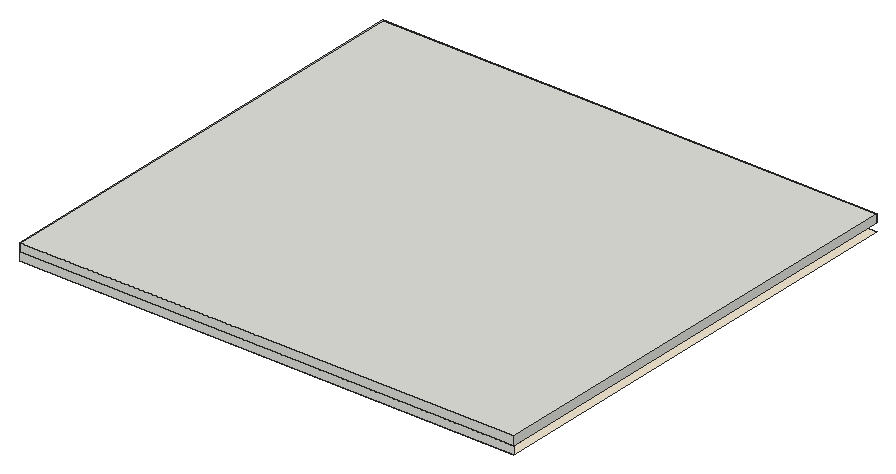
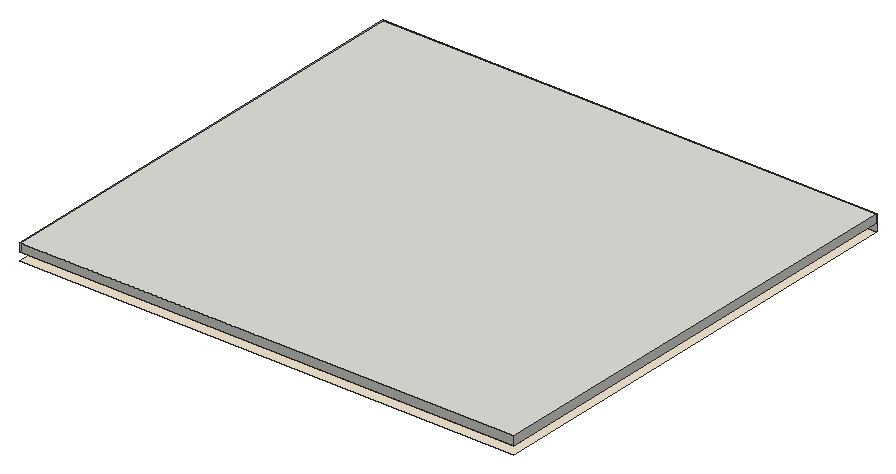
# SketchUp Ruby script. Lengths in inches.
U = 1.inch
M = Sketchup.active_model
def pt(a) = Geom::Point3d.new(a.map { |v| v * U })
def face(e, loops, mat)
  f = e.add_face(loops[0].map { |a| pt(a) })
  loops[1..].each { |l| e.add_face(l.map { |a| pt(a) }).erase! }
  f.material = f.back_material = mat if mat
  f
end
# faces: each face lists its corners as indices into pts; further lists are holes
def faces(e, pts, list, mat = nil) = list.each { |f| face(e, (f[0].is_a?(Array) ? f : [f]).map { |l| l.map { |i| pts[i] } }, mat) }
# xy, xz, yz: faces in a plane at the given z, y or x. An outline is a flat list of corners, or four numbers for a rectangle; further outlines are holes
def ring(l) = l.size == 4 ? [[l[0], l[1]], [l[2], l[1]], [l[2], l[3]], [l[0], l[3]]] : l.each_slice(2).to_a
def flat(e, list, mat, &to3) = list.each { |f| face(e, (f[0].is_a?(Array) ? f : [f]).map { |l| ring(l).map { |u, v| to3.(u, v) } }, mat) }
def xy(e, z, list, mat = nil) = flat(e, list, mat) { |x, y| [x, y, z] }
def xz(e, y, list, mat = nil) = flat(e, list, mat) { |x, z| [x, y, z] }
def yz(e, x, list, mat = nil) = flat(e, list, mat) { |y, z| [x, y, z] }
def lines(e, pts, list) = list.each { |a, b| e.add_line(pt(pts[a]), pt(pts[b])) }
# prism: a flat outline (further loops are holes) pulled along v
def prism(e, loops, v, mat = nil)
  f = face(e, loops, mat); d = Geom::Vector3d.new(v.map { |x| x * U })
  f.pushpull(f.normal.samedirection?(d) ? d.length : -d.length)
end
def box(e, o, s, mat = nil) = prism(e, [[o, [o[0] + s[0], o[1], o[2]], [o[0] + s[0], o[1] + s[1], o[2]], [o[0], o[1] + s[1], o[2]]]], [0, 0, s[2]], mat)
def at(x, y, z, deg = 0) = Geom::Transformation.translation(pt([x, y, z])) * Geom::Transformation.rotation(ORIGIN, Z_AXIS, deg.degrees)
def axes(o, x, y, z) = Geom::Transformation.new([*x, 0, *y, 0, *z, 0, *pt(o).to_a, 1])
def part(name) = M.definitions.add(name)
# library, detail: a bought-in or finely detailed component or shape, given as its bounding box
def library(name, o, s) = part(name).tap { |d| box(d.entities, o, s) }
def detail(e, o, s) = box(e.add_group.entities, o, s)
def put(e, d, t, mat = nil) = e.add_instance(d, t).tap { |i| i.material = mat if mat }
def group(e, t, mat = nil) = e.add_group.tap { |g| g.transformation = t; g.material = mat if mat }.entities
root = M.entities
M.materials.add("0961 AP 7892 PALE IVORY").color = [243, 232, 209]
xy(root,113.78,[[[12,0,198,171],[75.91,7.74,74.64,7.91,73.6,8.09,72.57,8.29,71.54,8.52,70.52,8.79,69.51,9.08,68.5,9.4,67.51,9.75,66.53,10.13,65.56,10.53,64.6,10.97,63.65,11.43,62.72,11.92,61.8,12.44,60.9,12.98,60.01,13.55,59.14,14.15,58.29,14.77,57.45,15.41,56.64,16.08,55.84,16.77,55.07,17.48,54.32,18.22,53.58,18.98,52.875,19.76,52.1875,20.56,51.52,21.375,50.88,22.21,50.27,23.07,49.68,23.9375,49.12,24.83,48.58,25.73,48.07,26.66,47.58,27.59,47.12,28.54,46.69,29.5,46.29,30.48,45.92,31.46,45.57,32.46,45.26,33.46,44.97,34.48,44.71,35.5,44.49,36.53,44.29,37.5625,44.12,38.6,43.99,39.65,43.88,40.69,43.8,41.74,43.76,42.8,43.74,43.82,43.74,129.03,43.76,130.04,43.8,131.07,43.88,132.1,43.99,133.13,44.13,134.16,44.3,135.18,44.5,136.2,44.74,137.21,45,138.21,45.29,139.2,45.61,140.18,45.97,141.16,46.35,142.12,46.76,143.07,47.2,144.01,47.66,144.93,48.16,145.84,48.68,146.74,49.23,147.62,49.8,148.48,50.41,149.32,51.03,150.15,51.68,150.95,52.36,151.74,53.05,152.5,53.77,153.25,54.52,153.97,55.28,154.67,56.07,155.34,56.87,156,57.7,156.62,58.54,157.22,59.4,157.8,60.28,158.35,61.17,158.875,62.08,159.37,63,159.84,63.94,160.28,64.89,160.69,65.85,161.07,66.83,161.43,67.81,161.75,68.8,162.05,69.8,162.31,70.8125,162.54,71.83,162.75,72.85,162.92,73.875,163.0625,74.9,163.17,76.04,163.26,158.18,163.26,159.32,163.16,160.35,163.05,161.37,162.9,162.38,162.72,163.39,162.51,164.39,162.27,165.39,162,166.375,161.7,167.35,161.375,168.32,161.02,169.28,160.63,170.22,160.22,171.15,159.77,172.07,159.3,172.97,158.8,173.86,158.28,174.73,157.73,175.59,157.15,176.42,156.54,177.24,155.92,178.04,155.26,178.82,154.59,179.58,153.89,180.3125,153.17,181.03,152.43,181.72,151.66,182.39,150.875,183.03,150.07,183.65,149.25,184.25,148.41,184.82,147.55,185.36,146.67,185.88,145.78,186.37,144.87,186.83,143.95,187.27,143.02,187.68,142.07,188.05,141.11,188.4,140.14,188.72,139.16,189.01,138.17,189.27,137.17,189.5,136.17,189.7,135.15,189.875,134.14,190.01,133.11,190.12,132.09,190.2,131.0625,190.24,130.03,190.26,129.03,190.26,42.89,190.24,41.88,190.2,40.84,190.12,39.8,190.02,38.77,189.88,37.74,189.71,36.71,189.51,35.69,189.29,34.68,189.03,33.67,188.74,32.67,188.42,31.68,188.08,30.7,187.7,29.73,187.3,28.77,186.87,27.82,186.41,26.89,185.93,25.97,185.42,25.0625,184.88,24.17,184.3125,23.3,183.72,22.44,183.11,21.61,182.47,20.79,181.8,19.98,181.12,19.2,180.41,18.44,179.68,17.7,178.92,16.99,178.15,16.29,177.36,15.62,176.54,14.97,175.71,14.35,174.86,13.75,173.99,13.17,173.11,12.625,172.21,12.1,171.3,11.61,170.37,11.14,169.43,10.7,168.47,10.29,167.51,9.9,166.53,9.55,165.54,9.22,164.54,8.92,163.54,8.65,162.53,8.41,161.51,8.21,160.48,8.03,159.45,7.88,158.24,7.74]],[[75.95,8.37,158.21,8.37,159.375,8.5,160.38,8.65,161.39,8.82,162.39,9.03,163.39,9.26,164.37,9.53,165.35,9.82,166.32,10.14,167.28,10.49,168.23,10.87,169.17,11.27,170.09,11.71,171,12.17,171.9,12.65,172.79,13.17,173.65,13.7,174.51,14.27,175.34,14.86,176.16,15.47,176.96,16.11,177.74,16.77,178.5,17.45,179.24,18.15,179.95,18.88,180.65,19.625,181.33,20.39,181.98,21.18,182.6,21.99,183.21,22.81,183.79,23.65,184.34,24.51,184.87,25.38,185.375,26.27,185.85,27.17,186.3,28.09,186.73,29.02,187.12,29.96,187.49,30.92,187.83,31.88,188.14,32.85,188.42,33.83,188.67,34.82,188.9,35.82,189.09,36.82,189.26,37.83,189.39,38.84,189.5,39.86,189.57,40.88,189.62,41.9,189.63,42.89,189.63,129.03,189.62,130.01,189.57,131.02,189.49,132.03,189.39,133.04,189.25,134.04,189.08,135.04,188.89,136.03,188.66,137.02,188.41,138,188.12,138.97,187.81,139.93,187.46,140.89,187.09,141.83,186.69,142.76,186.27,143.68,185.8125,144.58,185.33,145.47,184.82,146.35,184.29,147.21,183.73,148.05,183.15,148.875,182.54,149.68,181.9,150.47,181.25,151.25,180.57,152,179.86,152.72,179.14,153.43,178.4,154.12,177.63,154.78,176.85,155.42,176.05,156.04,175.22,156.63,174.39,157.2,173.53,157.74,172.66,158.26,171.77,158.74,170.87,159.21,169.96,159.64,169.03,160.05,168.09,160.43,167.14,160.78,166.19,161.1,165.22,161.4,164.24,161.66,163.25,161.9,162.26,162.1,161.27,162.28,160.26,162.42,159.26,162.54,158.15,162.63,76.0625,162.63,74.96,162.55,73.95,162.4375,72.94,162.3,71.94,162.13,70.95,161.93,69.95,161.7,68.97,161.4375,68,161.15,67.03,160.83,66.08,160.48,65.13,160.11,64.2,159.7,63.28,159.27,62.37,158.8125,61.48,158.33,60.6,157.8125,59.74,157.27,58.9,156.71,58.07,156.12,57.26,155.5,56.47,154.86,55.7,154.2,54.95,153.51,54.22,152.8,53.51,152.07,52.83,151.32,52.17,150.55,51.53,149.76,50.91,148.95,50.32,148.12,49.76,147.28,49.22,146.41,48.71,145.53,48.22,144.64,47.76,143.73,47.33,142.8125,46.93,141.88,46.56,140.93,46.21,139.98,45.89,139.01,45.61,138.04,45.35,137.05,45.12,136.0625,44.92,135.07,44.75,134.0625,44.62,133.06,44.51,132.05,44.43,131.03,44.39,130.02,44.37,129.03,44.37,43.82,44.39,42.82,44.43,41.78,44.51,40.75,44.61,39.72,44.75,38.69,44.91,37.67,45.1,36.65,45.33,35.64,45.58,34.64,45.86,33.64,46.17,32.65,46.51,31.68,46.88,30.71,47.27,29.75,47.69,28.81,48.14,27.87,48.62,26.95,49.125,26.05,49.65,25.16,50.21,24.28,50.79,23.43,51.39,22.59,52.02,21.76,52.67,20.96,53.35,20.17,54.04,19.41,54.76,18.66,55.5,17.94,56.26,17.24,57.05,16.56,57.85,15.9,58.67,15.27,59.5,14.66,60.36,14.08,61.23,13.52,62.12,12.98,63.02,12.48,63.93,11.99,64.86,11.54,65.81,11.11,66.76,10.71,67.73,10.34,68.7,10,69.69,9.68,70.69,9.39,71.6875,9.14,72.7,8.91,73.71,8.71,74.73,8.54],[76.02,9.37,74.88,9.53,73.89,9.69,72.9,9.88,71.92,10.11,70.95,10.36,69.98,10.64,69.02,10.94,68.07,11.28,67.14,11.64,66.21,12.03,65.29,12.44,64.39,12.89,63.5,13.35,62.62,13.85,61.76,14.37,60.91,14.91,60.08,15.48,59.27,16.07,58.47,16.6875,57.69,17.32,56.93,17.98,56.19,18.67,55.47,19.37,54.77,20.09,54.09,20.84,53.4375,21.6,52.81,22.38,52.19,23.18,51.61,24,51.04,24.83,50.5,25.68,49.99,26.55,49.5,27.43,49.04,28.32,48.6,29.23,48.19,30.15,47.81,31.08,47.45,32.02,47.12,32.97,46.82,33.93,46.55,34.9,46.3,35.87,46.08,36.85,45.89,37.84,45.74,38.84,45.6,39.83,45.5,40.84,45.43,41.84,45.39,42.84,45.37,43.83,45.37,129.02,45.39,129.99,45.43,130.97,45.5,131.96,45.61,132.9375,45.74,133.91,45.91,134.89,46.1,135.85,46.32,136.82,46.57,137.77,46.85,138.72,47.16,139.65,47.49,140.58,47.85,141.5,48.25,142.4,48.66,143.3,49.11,144.18,49.58,145.04,50.08,145.9,50.6,146.73,51.15,147.55,51.72,148.36,52.31,149.14,52.93,149.91,53.58,150.66,54.24,151.39,54.93,152.1,55.64,152.78,56.36,153.45,57.11,154.09,57.88,154.71,58.66,155.3125,59.47,155.88,60.28,156.43,61.12,156.96,61.97,157.46,62.84,157.93,63.72,158.375,64.61,158.79,65.52,159.19,66.43,159.55,67.36,159.89,68.3,160.2,69.24,160.48,70.2,160.73,71.16,160.95,72.125,161.14,73.1,161.31,74.07,161.44,75.05,161.55,76.1,161.63,158.11,161.63,159.16,161.54,160.14,161.43,161.11,161.29,162.08,161.12,163.04,160.92,163.99,160.69,164.94,160.44,165.88,160.15,166.8125,159.84,167.73,159.5,168.64,159.13,169.54,158.73,170.43,158.3125,171.3,157.86,172.16,157.39,173.01,156.89,173.84,156.36,174.65,155.8125,175.45,155.24,176.23,154.64,176.99,154.02,177.73,153.375,178.45,152.71,179.15,152.02,179.84,151.3125,180.49,150.58,181.13,149.84,181.75,149.07,182.34,148.29,182.9,147.48,183.45,146.67,183.97,145.83,184.46,144.98,184.93,144.12,185.37,143.24,185.78,142.35,186.17,141.45,186.53,140.53,186.86,139.61,187.17,138.68,187.44,137.73,187.69,136.78,187.91,135.83,188.1,134.86,188.26,133.89,188.39,132.92,188.5,131.94,188.57,130.96,188.62,129.98,188.63,129.02,188.63,42.9,188.62,41.93,188.57,40.9375,188.5,39.95,188.4,38.96,188.27,37.98,188.11,37,187.92,36.02,187.7,35.06,187.45,34.1,187.18,33.14,186.88,32.2,186.55,31.26,186.19,30.34,185.81,29.42,185.4,28.52,184.96,27.63,184.5,26.75,184.01,25.89,183.5,25.04,182.96,24.21,182.39,23.39,181.81,22.59,181.2,21.81,180.5625,21.04,179.91,20.3,179.23,19.57,178.54,18.87,177.82,18.18,177.08,17.52,176.32,16.88,175.55,16.26,174.75,15.67,173.94,15.09,173.11,14.55,172.27,14.02,171.41,13.53,170.54,13.05,169.66,12.61,168.76,12.1875,167.85,11.79,166.92,11.43,165.99,11.09,165.05,10.77,164.1,10.49,163.14,10.23,162.18,10.01,161.2,9.81,160.23,9.64,159.25,9.5,158.15,9.37]],[[76.09,10.37,158.09,10.37,159.12,10.49,160.07,10.625,161.02,10.79,161.96,10.98,162.9,11.2,163.83,11.45,164.75,11.73,165.66,12.03,166.57,12.36,167.46,12.72,168.35,13.1,169.22,13.51,170.08,13.9375,170.92,14.4,171.76,14.88,172.57,15.39,173.38,15.92,174.16,16.47,174.93,17.05,175.6875,17.65,176.42,18.27,177.14,18.92,177.83,19.58,178.51,20.27,179.17,20.97,179.8,21.69,180.42,22.43,181.01,23.19,181.58,23.97,182.125,24.76,182.65,25.57,183.15,26.39,183.62,27.23,184.07,28.08,184.49,28.95,184.89,29.82,185.26,30.71,185.61,31.61,185.93,32.52,186.22,33.43,186.49,34.36,186.73,35.29,186.9375,36.23,187.12,37.17,187.28,38.125,187.4,39.08,187.5,40.04,187.57,41,187.62,41.96,187.63,42.91,187.63,129.01,187.62,129.95,187.57,130.9,187.5,131.85,187.4,132.8,187.27,133.74,187.12,134.68,186.93,135.62,186.72,136.54,186.48,137.47,186.21,138.38,185.92,139.28,185.59,140.18,185.24,141.07,184.87,141.94,184.47,142.8,184.04,143.66,183.59,144.49,183.11,145.32,182.61,146.125,182.08,146.92,181.53,147.7,180.96,148.46,180.36,149.2,179.74,149.92,179.1,150.63,178.44,151.32,177.76,151.98,177.0625,152.63,176.34,153.25,175.61,153.85,174.85,154.43,174.08,154.99,173.29,155.52,172.49,156.03,171.67,156.52,170.83,156.98,169.99,157.41,169.125,157.82,168.25,158.21,167.37,158.5625,166.48,158.89,165.58,159.2,164.67,159.47,163.75,159.72,162.82,159.94,161.89,160.14,160.95,160.3,160.01,160.4375,159.0625,160.55,158.07,160.63,76.14,160.63,75.15,160.55,74.2,160.45,73.25,160.32,72.31,160.16,71.37,159.97,70.4375,159.76,69.51,159.51,68.59,159.24,67.6875,158.94,66.79,158.62,65.9,158.26,65.02,157.88,64.16,157.48,63.3,157.04,62.46,156.58,61.64,156.1,60.83,155.59,60.03,155.0625,59.26,154.51,58.49,153.93,57.75,153.33,57.03,152.7,56.32,152.06,55.64,151.39,54.97,150.7,54.33,150,53.7,149.27,53.1,148.53,52.52,147.76,51.97,146.99,51.4375,146.19,50.93,145.38,50.45,144.55,49.99,143.71,49.5625,142.86,49.16,141.99,48.78,141.12,48.43,140.23,48.1,139.33,47.8,138.42,47.53,137.5,47.29,136.58,47.08,135.64,46.89,134.71,46.73,133.76,46.6,132.82,46.5,131.86,46.43,130.91,46.39,129.96,46.37,129.01,46.37,43.84,46.39,42.875,46.43,41.9,46.5,40.92,46.6,39.95,46.72,38.98,46.88,38.02,47.0625,37.06,47.27,36.1,47.51,35.15,47.78,34.21,48.07,33.28,48.39,32.36,48.74,31.44,49.11,30.54,49.51,29.65,49.93,28.77,50.38,27.9,50.86,27.05,51.36,26.21,51.88,25.38,52.43,24.57,53,23.78,53.59,23,54.21,22.24,54.84,21.5,55.5,20.78,56.18,20.07,56.88,19.39,57.6,18.73,58.34,18.09,59.09,17.47,59.87,16.87,60.66,16.3,61.46,15.74,62.29,15.22,63.12,14.71,63.97,14.23,64.84,13.78,65.72,13.35,66.61,12.95,67.51,12.57,68.42,12.22,69.34,11.89,70.27,11.59,71.21,11.32,72.16,11.08,73.11,10.86,74.07,10.67,75.03,10.51],[76.16,11.37,75.18,11.5,74.25,11.66,73.32,11.84,72.39,12.05,71.48,12.29,70.5625,12.55,69.66,12.84,68.77,13.15,67.88,13.5,67.01,13.86,66.14,14.25,65.29,14.67,64.45,15.11,63.625,15.58,62.8125,16.07,62.02,16.58,61.23,17.11,60.47,17.67,59.71,18.25,58.98,18.85,58.27,19.47,57.57,20.12,56.89,20.78,56.23,21.46,55.59,22.16,54.97,22.88,54.375,23.62,53.8,24.37,53.25,25.14,52.72,25.93,52.21,26.73,51.72,27.54,51.26,28.37,50.83,29.21,50.42,30.07,50.03,30.93,49.67,31.8125,49.33,32.7,49.02,33.59,48.74,34.5,48.48,35.41,48.25,36.33,48.04,37.26,47.86,38.1875,47.71,39.125,47.59,40.07,47.49,41.01,47.43,41.95,47.39,42.9,47.37,43.85,47.37,129,47.39,129.93,47.43,130.85,47.5,131.77,47.59,132.7,47.72,133.61,47.875,134.53,48.05,135.43,48.26,136.34,48.5,137.23,48.76,138.12,49.05,139,49.36,139.87,49.7,140.73,50.07,141.58,50.46,142.42,50.88,143.25,51.32,144.0625,51.79,144.86,52.28,145.65,52.79,146.42,53.33,147.17,53.89,147.91,54.47,148.63,55.07,149.33,55.7,150.02,56.34,150.68,57.01,151.33,57.69,151.95,58.39,152.56,59.11,153.14,59.85,153.7,60.6,154.24,61.37,154.75,62.16,155.25,62.96,155.71,63.77,156.16,64.6,156.58,65.43,156.97,66.28,157.34,67.14,157.68,68.01,158,68.89,158.29,69.78,158.55,70.68,158.79,71.58,159,72.49,159.18,73.4,159.33,74.32,159.46,75.24,159.56,76.18,159.63,158.03,159.63,158.96,159.55,159.88,159.45,160.79,159.3125,161.7,159.15,162.6,158.97,163.5,158.75,164.39,158.51,165.27,158.25,166.15,157.95,167.01,157.63,167.87,157.29,168.71,156.91,169.54,156.52,170.36,156.1,171.17,155.65,171.96,155.18,172.74,154.6875,173.51,154.17,174.25,153.63,174.99,153.07,175.7,152.49,176.4,151.88,177.07,151.26,177.73,150.61,178.375,149.95,178.99,149.26,179.59,148.5625,180.17,147.84,180.72,147.11,181.25,146.35,181.76,145.59,182.25,144.8,182.71,144,183.15,143.19,183.57,142.37,183.96,141.53,184.32,140.6875,184.66,139.83,184.97,138.96,185.26,138.08,185.51,137.2,185.75,136.31,185.95,135.41,186.13,134.5,186.28,133.59,186.41,132.68,186.51,131.76,186.57,130.84,186.62,129.92,186.63,129,186.63,42.92,186.62,41.99,186.58,41.06,186.51,40.125,186.41,39.2,186.29,38.27,186.14,37.35,185.96,36.43,185.76,35.52,185.52,34.62,185.27,33.72,184.98,32.83,184.67,31.95,184.34,31.08,183.98,30.22,183.59,29.375,183.18,28.54,182.74,27.71,182.28,26.9,181.8,26.1,181.29,25.32,180.76,24.55,180.21,23.8,179.64,23.06,179.04,22.34,178.43,21.64,177.79,20.96,177.13,20.29,176.46,19.65,175.76,19.03,175.05,18.42,174.32,17.84,173.58,17.28,172.8125,16.75,172.04,16.23,171.24,15.74,170.44,15.27,169.61,14.83,168.78,14.41,167.9375,14.01,167.08,13.64,166.21,13.29,165.34,12.98,164.45,12.68,163.56,12.41,162.65,12.17,161.75,11.96,160.83,11.77,159.91,11.61,158.99,11.48,158.04,11.37]]],"0961 AP 7892 PALE IVORY")
xy(root,116.78,[[12,0,198,171]],"0961 AP 7892 PALE IVORY")
xy(root,120,[[12,0,198,171]])
xz(root,0,[[12,113.78,198,116.78],[12,116.78,198,120]])
xz(root,11.37,[[76.16,113.78,158.04,115.78]],"0961 AP 7892 PALE IVORY")
xz(root,159.63,[[76.18,113.78,158.03,115.78]],"0961 AP 7892 PALE IVORY")
xz(root,171,[[12,116.78,198,120]])
yz(root,12,[[0,116.78,171,120]])
yz(root,47.37,[[43.85,113.78,129,115.78]],"0961 AP 7892 PALE IVORY")
yz(root,186.63,[[42.92,113.78,129,115.78]],"0961 AP 7892 PALE IVORY")
yz(root,198,[[0,116.78,171,120]])
p = [[54.87,24.01,113.3125],[54.31,24.75,113.3125],[54.31,24.75,115.78],[54.87,24.01,115.78],[53.76,25.5,113.3125],[53.76,25.5,115.78],
  [53.24,26.27,113.3125],[53.24,26.27,115.78],[52.75,27.06,113.3125],[52.75,27.06,115.78],[52.27,27.86,113.3125],[52.27,27.86,115.78],
  [51.82,28.67,113.3125],[51.82,28.67,115.78],[51.39,29.5,113.3125],[51.39,29.5,115.78],[50.99,30.33,113.3125],[50.99,30.33,115.78],
  [50.61,31.18,113.3125],[50.61,31.18,115.78],[50.25,32.04,113.3125],[50.25,32.04,115.78],[49.92,32.91,113.3125],[49.92,32.91,115.78],
  [49.62,33.79,113.3125],[49.62,33.79,115.78],[49.34,34.68,113.3125],[49.34,34.68,115.78],[49.09,35.57,113.3125],[49.09,35.57,115.78],
  [48.86,36.48,113.3125],[48.86,36.48,115.78],[48.66,37.38,113.3125],[48.66,37.38,115.78],[48.49,38.3,113.3125],[48.49,38.3,115.78],
  [48.34,39.22,113.3125],[48.34,39.22,115.78],[48.22,40.14,113.3125],[48.22,40.14,115.78],[48.12,41.0625,113.3125],[48.12,41.0625,115.78],
  [48.06,41.99,113.3125],[48.06,41.99,115.78],[48.01,42.92,113.3125],[48.01,42.92,115.78],[48,43.85,113.3125],[48,43.85,115.78],
  [75.18,11.5,113.78],[76.16,11.37,113.78],[76.16,11.37,115.78],[75.18,11.5,115.78],[158.04,11.37,113.78],[158.99,11.48,113.78],
  [158.99,11.48,115.78],[158.04,11.37,115.78],[74.25,11.66,113.78],[74.25,11.66,115.78],[159.91,11.61,113.78],[159.91,11.61,115.78],
  [160.83,11.77,113.78],[160.83,11.77,115.78],[73.32,11.84,113.78],[73.32,11.84,115.78],[72.39,12.05,113.78],[72.39,12.05,115.78],
  [161.75,11.96,113.78],[161.75,11.96,115.78],[162.65,12.17,113.78],[162.65,12.17,115.78],[71.48,12.29,113.78],[71.48,12.29,115.78],
  [163.56,12.41,113.78],[163.56,12.41,115.78],[70.5625,12.55,113.78],[70.5625,12.55,115.78],[164.45,12.68,113.78],[164.45,12.68,115.78],
  [69.66,12.84,113.78],[69.66,12.84,115.78],[165.34,12.98,113.78],[165.34,12.98,115.78],[68.77,13.15,113.78],[68.77,13.15,115.78],
  [166.21,13.29,113.78],[166.21,13.29,115.78],[67.88,13.5,113.78],[67.88,13.5,115.78],[167.08,13.64,113.78],[167.08,13.64,115.78],
  [67.01,13.86,113.78],[67.01,13.86,115.78],[167.9375,14.01,113.78],[167.9375,14.01,115.78],[66.14,14.25,113.78],[66.14,14.25,115.78],
  [168.78,14.41,113.78],[168.78,14.41,115.78],[65.29,14.67,113.78],[65.29,14.67,115.78],[169.61,14.83,113.78],[169.61,14.83,115.78],
  [64.45,15.11,113.78],[64.45,15.11,115.78],[170.44,15.27,113.78],[170.44,15.27,115.78],[63.625,15.58,113.78],[63.625,15.58,115.78],
  [171.24,15.74,113.78],[171.24,15.74,115.78],[62.8125,16.07,113.78],[62.8125,16.07,115.78],[172.04,16.23,113.78],[172.04,16.23,115.78],
  [62.02,16.58,113.78],[62.02,16.58,115.78],[172.8125,16.75,113.78],[172.8125,16.75,115.78],[61.23,17.11,113.78],[61.23,17.11,115.78],
  [173.58,17.28,113.78],[173.58,17.28,115.78],[60.47,17.67,113.78],[60.47,17.67,115.78],[174.32,17.84,113.78],[174.32,17.84,115.78],
  [59.71,18.25,113.78],[59.71,18.25,115.78],[175.05,18.42,113.78],[175.05,18.42,115.78],[58.98,18.85,113.78],[58.98,18.85,115.78],
  [175.76,19.03,113.78],[175.76,19.03,115.78],[58.27,19.47,113.78],[58.27,19.47,115.78],[176.46,19.65,113.78],[176.46,19.65,115.78],
  [57.57,20.12,113.78],[57.57,20.12,115.78],[177.13,20.29,113.78],[177.13,20.29,115.78],[56.89,20.78,113.78],[56.89,20.78,115.78],
  [177.79,20.96,113.78],[177.79,20.96,115.78],[56.23,21.46,113.78],[56.23,21.46,115.78],[178.43,21.64,113.78],[178.43,21.64,115.78],
  [55.59,22.16,113.78],[55.59,22.16,115.78],[179.04,22.34,113.78],[179.04,22.34,115.78],[54.97,22.88,113.78],[54.97,22.88,115.78],
  [179.64,23.06,113.78],[179.64,23.06,115.78],[54.375,23.62,113.78],[54.375,23.62,115.78],[180.21,23.8,113.78],[180.21,23.8,115.78],
  [53.8,24.37,113.78],[53.8,24.37,115.78],[180.76,24.55,113.78],[180.76,24.55,115.78],[53.25,25.14,113.78],[53.25,25.14,115.78],
  [181.29,25.32,113.78],[181.29,25.32,115.78],[52.72,25.93,113.78],[52.72,25.93,115.78],[181.8,26.1,113.78],[181.8,26.1,115.78],
  [52.21,26.73,113.78],[52.21,26.73,115.78],[182.28,26.9,113.78],[182.28,26.9,115.78],[51.72,27.54,113.78],[51.72,27.54,115.78],
  [182.74,27.71,113.78],[182.74,27.71,115.78],[51.26,28.37,113.78],[51.26,28.37,115.78],[183.18,28.54,113.78],[183.18,28.54,115.78],
  [50.83,29.21,113.78],[50.83,29.21,115.78],[183.59,29.375,113.78],[183.59,29.375,115.78],[50.42,30.07,113.78],[50.42,30.07,115.78],
  [183.98,30.22,113.78],[183.98,30.22,115.78],[50.03,30.93,113.78],[50.03,30.93,115.78],[184.34,31.08,113.78],[184.34,31.08,115.78],
  [49.67,31.8125,113.78],[49.67,31.8125,115.78],[184.67,31.95,113.78],[184.67,31.95,115.78],[49.33,32.7,113.78],[49.33,32.7,115.78],
  [184.98,32.83,113.78],[184.98,32.83,115.78],[49.02,33.59,113.78],[49.02,33.59,115.78],[185.27,33.72,113.78],[185.27,33.72,115.78],
  [48.74,34.5,113.78],[48.74,34.5,115.78],[185.52,34.62,113.78],[185.52,34.62,115.78],[48.48,35.41,113.78],[48.48,35.41,115.78],
  [185.76,35.52,113.78],[185.76,35.52,115.78],[48.25,36.33,113.78],[48.25,36.33,115.78],[185.96,36.43,113.78],[185.96,36.43,115.78],
  [48.04,37.26,113.78],[48.04,37.26,115.78],[186.14,37.35,113.78],[186.14,37.35,115.78],[47.86,38.1875,113.78],[47.86,38.1875,115.78],
  [186.29,38.27,113.78],[186.29,38.27,115.78],[47.71,39.125,113.78],[47.71,39.125,115.78],[186.41,39.2,113.78],[186.41,39.2,115.78],
  [47.59,40.07,113.78],[47.59,40.07,115.78],[186.51,40.125,113.78],[186.51,40.125,115.78],[47.49,41.01,113.78],[47.49,41.01,115.78],
  [186.58,41.06,113.78],[186.58,41.06,115.78],[47.43,41.95,113.78],[47.43,41.95,115.78],[186.62,41.99,113.78],[186.62,41.99,115.78],
  [47.39,42.9,113.78],[47.39,42.9,115.78],[186.63,42.92,113.78],[186.63,42.92,115.78],[47.37,43.85,113.78],[47.37,43.85,115.78],
  [47.39,129.93,113.78],[47.37,129,113.78],[47.37,129,115.78],[47.39,129.93,115.78],[186.63,129,113.78],[186.62,129.92,113.78],
  [186.62,129.92,115.78],[186.63,129,115.78],[47.43,130.85,113.78],[47.43,130.85,115.78],[186.57,130.84,113.78],[186.57,130.84,115.78],
  [186.51,131.76,113.78],[186.51,131.76,115.78],[47.5,131.77,113.78],[47.5,131.77,115.78],[47.59,132.7,113.78],[47.59,132.7,115.78],
  [186.41,132.68,113.78],[186.41,132.68,115.78],[47.72,133.61,113.78],[47.72,133.61,115.78],[186.28,133.59,113.78],[186.28,133.59,115.78],
  [47.875,134.53,113.78],[47.875,134.53,115.78],[186.13,134.5,113.78],[186.13,134.5,115.78],[48.05,135.43,113.78],[48.05,135.43,115.78],
  [185.95,135.41,113.78],[185.95,135.41,115.78],[48.26,136.34,113.78],[48.26,136.34,115.78],[185.75,136.31,113.78],[185.75,136.31,115.78],
  [48.5,137.23,113.78],[48.5,137.23,115.78],[185.51,137.2,113.78],[185.51,137.2,115.78],[48.76,138.12,113.78],[48.76,138.12,115.78],
  [185.26,138.08,113.78],[185.26,138.08,115.78],[49.05,139,113.78],[49.05,139,115.78],[184.97,138.96,113.78],[184.97,138.96,115.78],
  [49.36,139.87,113.78],[49.36,139.87,115.78],[49.7,140.73,113.78],[49.7,140.73,115.78],[50.07,141.58,113.78],[50.07,141.58,115.78],
  [50.46,142.42,113.78],[50.46,142.42,115.78],[50.88,143.25,113.78],[50.88,143.25,115.78],[51.32,144.0625,113.78],[51.32,144.0625,115.78],
  [51.79,144.86,113.78],[51.79,144.86,115.78],[52.28,145.65,113.78],[52.28,145.65,115.78],[52.79,146.42,113.78],[52.79,146.42,115.78],
  [53.33,147.17,113.78],[53.33,147.17,115.78],[53.89,147.91,113.78],[53.89,147.91,115.78],[54.47,148.63,113.78],[54.47,148.63,115.78],
  [55.07,149.33,113.78],[55.07,149.33,115.78],[55.7,150.02,113.78],[55.7,150.02,115.78],[56.34,150.68,113.78],[56.34,150.68,115.78],
  [57.01,151.33,113.78],[57.01,151.33,115.78],[57.69,151.95,113.78],[57.69,151.95,115.78],[176.4,151.88,113.78],[175.7,152.49,113.78],
  [175.7,152.49,115.78],[176.4,151.88,115.78],[58.39,152.56,113.78],[58.39,152.56,115.78],[174.99,153.07,113.78],[174.99,153.07,115.78],
  [59.11,153.14,113.78],[59.11,153.14,115.78],[59.85,153.7,113.78],[59.85,153.7,115.78],[174.25,153.63,113.78],[174.25,153.63,115.78],
  [173.51,154.17,113.78],[173.51,154.17,115.78],[60.6,154.24,113.78],[60.6,154.24,115.78],[61.37,154.75,113.78],[61.37,154.75,115.78],
  [172.74,154.6875,113.78],[172.74,154.6875,115.78],[171.96,155.18,113.78],[171.96,155.18,115.78],[62.16,155.25,113.78],[62.16,155.25,115.78],
  [62.96,155.71,113.78],[62.96,155.71,115.78],[171.17,155.65,113.78],[171.17,155.65,115.78],[63.77,156.16,113.78],[63.77,156.16,115.78],
  [170.36,156.1,113.78],[170.36,156.1,115.78],[169.54,156.52,113.78],[169.54,156.52,115.78],[64.6,156.58,113.78],[64.6,156.58,115.78],
  [168.71,156.91,113.78],[168.71,156.91,115.78],[65.43,156.97,113.78],[65.43,156.97,115.78],[167.87,157.29,113.78],[167.87,157.29,115.78],
  [66.28,157.34,113.78],[66.28,157.34,115.78],[67.14,157.68,113.78],[67.14,157.68,115.78],[167.01,157.63,113.78],[167.01,157.63,115.78],
  [166.15,157.95,113.78],[166.15,157.95,115.78],[68.01,158,113.78],[68.01,158,115.78],[68.89,158.29,113.78],[68.89,158.29,115.78],
  [165.27,158.25,113.78],[165.27,158.25,115.78],[164.39,158.51,113.78],[164.39,158.51,115.78],[69.78,158.55,113.78],[69.78,158.55,115.78],
  [163.5,158.75,113.78],[163.5,158.75,115.78],[70.68,158.79,113.78],[70.68,158.79,115.78],[71.58,159,113.78],[71.58,159,115.78],
  [162.6,158.97,113.78],[162.6,158.97,115.78],[72.49,159.18,113.78],[72.49,159.18,115.78],[161.7,159.15,113.78],[161.7,159.15,115.78],
  [73.4,159.33,113.78],[73.4,159.33,115.78],[160.79,159.3125,113.78],[160.79,159.3125,115.78],[74.32,159.46,113.78],[74.32,159.46,115.78],
  [159.88,159.45,113.78],[159.88,159.45,115.78],[158.96,159.55,113.78],[158.96,159.55,115.78],[75.24,159.56,113.78],[75.24,159.56,115.78],
  [76.18,159.63,113.78],[76.18,159.63,115.78],[158.03,159.63,113.78],[158.03,159.63,115.78]]
faces(root,p,[[0,1,2,3],[1,4,5,2],[4,6,7,5],[6,8,9,7],[8,10,11,9],[10,12,13,11],[12,14,15,13],[14,16,17,15],
  [16,18,19,17],[18,20,21,19],[20,22,23,21],[22,24,25,23],[24,26,27,25],[26,28,29,27],[28,30,31,29],[30,32,33,31],
  [32,34,35,33],[34,36,37,35],[36,38,39,37],[38,40,41,39],[40,42,43,41],[42,44,45,43],[44,46,47,45],[48,49,50,51],
  [52,53,54,55],[56,48,51,57],[53,58,59,54],[58,60,61,59],[62,56,57,63],[64,62,63,65],[60,66,67,61],[66,68,69,67],
  [70,64,65,71],[68,72,73,69],[74,70,71,75],[72,76,77,73],[78,74,75,79],[76,80,81,77],[82,78,79,83],[80,84,85,81],
  [86,82,83,87],[84,88,89,85],[90,86,87,91],[88,92,93,89],[94,90,91,95],[92,96,97,93],[98,94,95,99],[96,100,101,97],
  [102,98,99,103],[100,104,105,101],[106,102,103,107],[104,108,109,105],[110,106,107,111],[108,112,113,109],[114,110,111,115],[112,116,117,113],
  [118,114,115,119],[116,120,121,117],[122,118,119,123],[120,124,125,121],[126,122,123,127],[124,128,129,125],[130,126,127,131],[128,132,133,129],
  [134,130,131,135],[132,136,137,133],[138,134,135,139],[136,140,141,137],[142,138,139,143],[140,144,145,141],[146,142,143,147],[144,148,149,145],
  [150,146,147,151],[148,152,153,149],[154,150,151,155],[152,156,157,153],[158,154,155,159],[156,160,161,157],[162,158,159,163],[160,164,165,161],
  [166,162,163,167],[164,168,169,165],[170,166,167,171],[168,172,173,169],[174,170,171,175],[172,176,177,173],[178,174,175,179],[176,180,181,177],
  [182,178,179,183],[180,184,185,181],[186,182,183,187],[184,188,189,185],[190,186,187,191],[188,192,193,189],[194,190,191,195],[192,196,197,193],
  [198,194,195,199],[196,200,201,197],[202,198,199,203],[200,204,205,201],[206,202,203,207],[204,208,209,205],[210,206,207,211],[208,212,213,209],
  [214,210,211,215],[212,216,217,213],[218,214,215,219],[216,220,221,217],[222,218,219,223],[220,224,225,221],[226,222,223,227],[224,228,229,225],
  [230,226,227,231],[228,232,233,229],[234,230,231,235],[232,236,237,233],[238,234,235,239],[236,240,241,237],[242,238,239,243],[240,244,245,241],
  [246,242,243,247],[244,248,249,245],[250,246,247,251],[252,253,254,255],[256,257,258,259],[260,252,255,261],[257,262,263,258],[262,264,265,263],
  [266,260,261,267],[268,266,267,269],[264,270,271,265],[272,268,269,273],[270,274,275,271],[276,272,273,277],[274,278,279,275],[280,276,277,281],
  [278,282,283,279],[284,280,281,285],[282,286,287,283],[288,284,285,289],[286,290,291,287],[292,288,289,293],[290,294,295,291],[296,292,293,297],
  [294,298,299,295],[300,296,297,301],[302,300,301,303],[304,302,303,305],[306,304,305,307],[308,306,307,309],[310,308,309,311],[312,310,311,313],
  [314,312,313,315],[316,314,315,317],[318,316,317,319],[320,318,319,321],[322,320,321,323],[324,322,323,325],[326,324,325,327],[328,326,327,329],
  [330,328,329,331],[332,330,331,333],[334,335,336,337],[338,332,333,339],[335,340,341,336],[342,338,339,343],[344,342,343,345],[340,346,347,341],
  [346,348,349,347],[350,344,345,351],[352,350,351,353],[348,354,355,349],[354,356,357,355],[358,352,353,359],[360,358,359,361],[356,362,363,357],
  [364,360,361,365],[362,366,367,363],[366,368,369,367],[370,364,365,371],[368,372,373,369],[374,370,371,375],[372,376,377,373],[378,374,375,379],
  [380,378,379,381],[376,382,383,377],[382,384,385,383],[386,380,381,387],[388,386,387,389],[384,390,391,385],[390,392,393,391],[394,388,389,395],
  [392,396,397,393],[398,394,395,399],[400,398,399,401],[396,402,403,397],[404,400,401,405],[402,406,407,403],[408,404,405,409],[406,410,411,407],
  [412,408,409,413],[410,414,415,411],[414,416,417,415],[418,412,413,419],[420,418,419,421],[416,422,423,417]],"0961 AP 7892 PALE IVORY")
